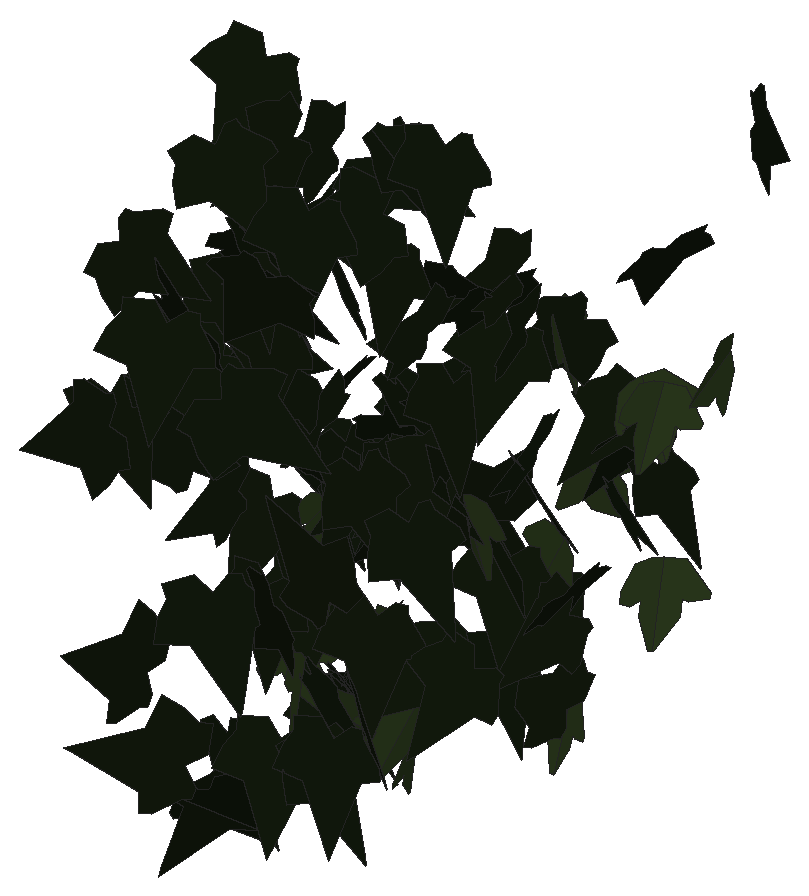
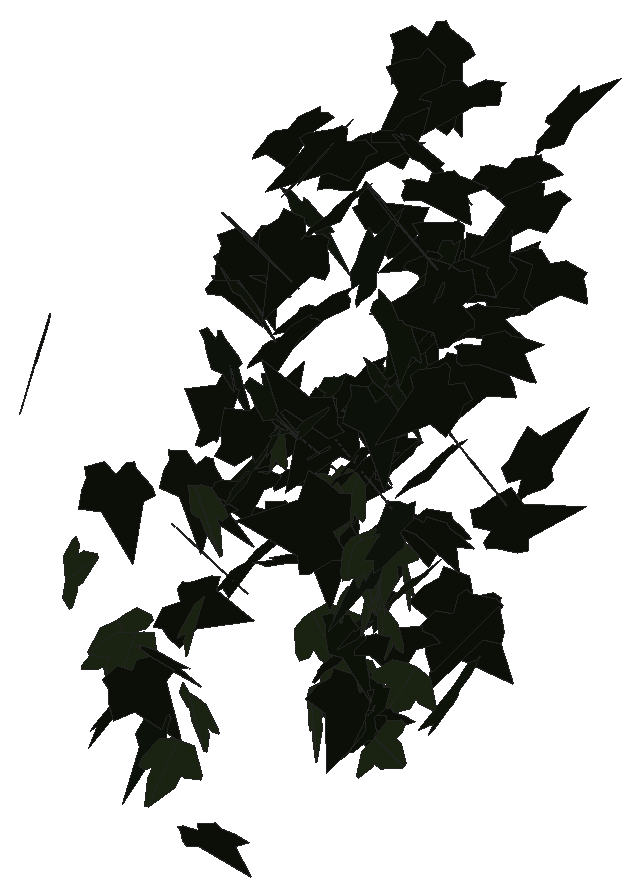
# SketchUp Ruby script. Lengths in inches.
U = 1.inch
M = Sketchup.active_model
def pt(a) = Geom::Point3d.new(a.map { |v| v * U })
def face(e, loops, mat)
  f = e.add_face(loops[0].map { |a| pt(a) })
  loops[1..].each { |l| e.add_face(l.map { |a| pt(a) }).erase! }
  f.material = f.back_material = mat if mat
  f
end
# faces: each face lists its corners as indices into pts; further lists are holes
def faces(e, pts, list, mat = nil) = list.each { |f| face(e, (f[0].is_a?(Array) ? f : [f]).map { |l| l.map { |i| pts[i] } }, mat) }
# xy, xz, yz: faces in a plane at the given z, y or x. An outline is a flat list of corners, or four numbers for a rectangle; further outlines are holes
def ring(l) = l.size == 4 ? [[l[0], l[1]], [l[2], l[1]], [l[2], l[3]], [l[0], l[3]]] : l.each_slice(2).to_a
def flat(e, list, mat, &to3) = list.each { |f| face(e, (f[0].is_a?(Array) ? f : [f]).map { |l| ring(l).map { |u, v| to3.(u, v) } }, mat) }
def xy(e, z, list, mat = nil) = flat(e, list, mat) { |x, y| [x, y, z] }
def xz(e, y, list, mat = nil) = flat(e, list, mat) { |x, z| [x, y, z] }
def yz(e, x, list, mat = nil) = flat(e, list, mat) { |y, z| [x, y, z] }
def lines(e, pts, list) = list.each { |a, b| e.add_line(pt(pts[a]), pt(pts[b])) }
# prism: a flat outline (further loops are holes) pulled along v
def prism(e, loops, v, mat = nil)
  f = face(e, loops, mat); d = Geom::Vector3d.new(v.map { |x| x * U })
  f.pushpull(f.normal.samedirection?(d) ? d.length : -d.length)
end
def box(e, o, s, mat = nil) = prism(e, [[o, [o[0] + s[0], o[1], o[2]], [o[0] + s[0], o[1] + s[1], o[2]], [o[0], o[1] + s[1], o[2]]]], [0, 0, s[2]], mat)
def at(x, y, z, deg = 0) = Geom::Transformation.translation(pt([x, y, z])) * Geom::Transformation.rotation(ORIGIN, Z_AXIS, deg.degrees)
def axes(o, x, y, z) = Geom::Transformation.new([*x, 0, *y, 0, *z, 0, *pt(o).to_a, 1])
def part(name) = M.definitions.add(name)
# library, detail: a bought-in or finely detailed component or shape, given as its bounding box
def library(name, o, s) = part(name).tap { |d| box(d.entities, o, s) }
def detail(e, o, s) = box(e.add_group.entities, o, s)
def put(e, d, t, mat = nil) = e.add_instance(d, t).tap { |i| i.material = mat if mat }
def group(e, t, mat = nil) = e.add_group.tap { |g| g.transformation = t; g.material = mat if mat }.entities
root = M.entities
M.materials.add("efeu1").color = [18, 25, 13]
M.materials.add("efeu2").color = [43, 57, 29]
c1 = part("ivyleaf_9")
p = [[1.54,2.16,1.25],[1.36,2.04,1.19],[-0.21,0.99,0.68],[-0.71,1.11,0.82],[-0.85,0.86,0.67],[-0.8,0.17,0.21],
  [-0.9,-0.01,0.1],[-0.67,-0.16,-0.02],[-0.08,-0.08,-0.05],[-0.03,-0.6,-0.4],[0.65,-0.88,-0.66],[0.83,-0.6,-0.49],
  [1.29,-0.42,-0.43],[1.8125,-0.07,-0.26],[1.21,0.44,0.15]]
faces(c1.entities,p,[[0,1,2,3,4,5,6,7,8,9,10,11,12,13,14]],"efeu1")
c2 = part("ivyleaf_10")
p = [[0,0.5,-0.03],[-0.0625,2.02,-0.43],[-0.19,2.01,-0.46],[-0.54,1.05,-0.29],[-0.52,0.625,-0.18],[-0.83,0.76,-0.28],
  [-1.16,0.64,-0.33],[-1.15,0.33,-0.24],[-0.77,-0.39,0.02],[-0.3,-0.51,0.16],[0.04,-0.48,0.23],[-0.02,2.01,-0.4375],
  [-0.06,2.01,-0.43],[0.04,-0.49,0.23],[0.67,-0.49,0.14],[1.38,0.36,-0.2],[1.375,0.51,-0.24],[0.81,0.65,-0.19],
  [0.62,0.59,-0.15],[0.6,1.09,-0.28],[0.5,1.23,-0.31]]
faces(c2.entities,p,[[0,1,2,3,4,5,6,7,8,9,10],[11,12,0,13,14,15,16,17,18,19,20]],"efeu2")
put(root,c1,axes([629.85,118.33,320.14],[-1.05111,-0.93043,0.08005],[-0.05037,-0.06385,-1.40368],[0.93251,-1.05222,0.0144]))
put(root,c1,axes([629.95,121.9,329.74],[-0.98839,-0.8944,-0.09871],[0.06806,0.0719,-1.33297],[0.89725,-0.9907,-0.00762]))
put(root,c2,axes([629.7,123.79,306.15],[-1.03186,-0.37718,-0.54841],[0.62092,-0.18105,-1.04376],[0.23975,-1.15443,0.34287]))
put(root,c2,axes([630.0625,125.32,303.48],[0.25648,0.92168,-0.76849],[-0.25719,-0.72537,-0.95579],[-1.17215,0.36083,0.04156]))
put(root,c1,axes([629.92,124.72,308.45],[-0.52487,-1.07341,-0.35701],[0.17536,0.3116,-1.1947],[1.11755,-0.55303,0.0198]))
put(root,c1,axes([630.25,121.9,312.72],[-1.12203,-0.49957,-0.40756],[0.40329,0.09442,-1.226],[0.50303,-1.19002,0.07382]))
put(root,c1,axes([629.7,124.1,310.51],[-0.03949,-1.15836,0.48367],[0.26125,-0.4809,-1.13039],[1.2278,0.06507,0.25608]))
put(root,c1,axes([629.79,114.55,325.82],[0.38981,-0.4459,-1.19635],[-0.12214,1.2321,-0.49902],[1.27089,0.25517,0.31899]))
put(root,c1,axes([630.09,120.75,319.09],[0.16006,0.06924,-1.32906],[-0.32833,1.29931,0.02815],[1.28972,0.32218,0.1721]))
put(root,c1,axes([630.9375,122.96,322.99],[-0.20763,1.04748,0.75387],[-0.20421,0.72728,-1.06677],[-1.2743,-0.28722,0.04812]))
put(root,c1,axes([629.64,120.48,304.03],[0.82578,-1.15992,-0.03923],[-0.02272,0.03198,-1.42384],[1.16036,0.82609,0.00004]))
put(root,c1,axes([629.7,120.33,323.08],[0.87461,0.16047,0.98959],[0.83483,0.61055,-0.83683],[-0.55508,1.1711,0.30068]))
put(root,c2,axes([630.15,124.75,309.44],[1.06337,-0.50755,0.41179],[0.44059,-0.02421,-1.16758],[0.48276,1.14006,0.15854]))
put(root,c1,axes([630.91,136.59,303.67],[-1.12475,-0.4794,-0.04315],[0.03909,0.01833,-1.22266],[0.47975,-1.12543,-0.00153]))
put(root,c1,axes([631.46,118.46,315.09],[-1.13617,0.55762,0.10034],[-0.07939,0.06594,-1.2654],[-0.56099,-1.13868,-0.02415]))
put(root,c2,axes([631.16,124.11,312.08],[-0.66363,-1.0746,0.04055],[-0.0351,-0.02598,-1.2629],[1.07479,-0.66436,-0.0162]))
put(root,c1,axes([631.39,117.6875,320.6],[-0.98385,-0.80675,0.37955],[-0.27516,-0.26289,-1.27202],[0.84805,-1.02123,0.02761]))
put(root,c1,axes([630.22,123.89,313.17],[1.06374,-0.68486,0.17281],[0.28329,0.12751,-1.23852],[0.64703,1.07011,0.25817]))
put(root,c2,axes([631.31,124.14,310.46],[-0.9243,0.82505,0.09608],[-0.06849,0.06756,-1.23896],[-0.8278,-0.92682,-0.00478]))
put(root,c1,axes([631.24,124.95,304.01],[-0.66697,-1.02849,-0.18823],[0.13194,0.13869,-1.22533],[1.03722,-0.679,0.03483]))
put(root,c1,axes([631.21,124.12,311.6],[1.05332,-0.1652,-0.6635],[-0.56826,0.46619,-1.01821],[0.38026,1.15428,0.31627]))
put(root,c1,axes([631.51,116.1,322.09],[0.94752,-0.72708,0.58664],[-0.3929,0.44794,1.18977],[-0.8476,-1.02043,0.10428]))
put(root,c1,axes([630.55,125.26,304.54],[0.8076,-0.6856,0.62738],[0.50223,-0.37735,-1.05889],[0.78193,0.95049,0.03215]))
put(root,c1,axes([630.96,112.43,321.17],[-0.5158,-0.64825,-1.06719],[0.73295,0.77762,-0.8266],[1.0109,-0.89457,0.05481]))
put(root,c1,axes([631.53,125,305.17],[0.71702,1.00502,-0.03351],[-0.02036,-0.02664,-1.23458],[-1.00538,0.7173,0.0011]))
put(root,c2,axes([631.74,124.39,312.07],[-0.30232,-1.21917,0.07984],[-0.00639,-0.08067,-1.25603],[1.22177,-0.3021,0.01319]))
put(root,c1,axes([631.92,112.98,310.69],[-0.07155,-0.07773,1.43345],[-0.90642,-1.1105,-0.10546],[1.1132,-0.90922,0.00626]))
put(root,c1,axes([630.89,120.05,323.92],[1.00123,-1.01155,0.16192],[0.10518,-0.12371,-1.42321],[1.01901,1.00667,-0.01219]))
put(root,c1,axes([631.0625,125.2,304.2],[0.80695,-0.89437,0.2562],[0.1472,-0.21213,-1.20417],[0.91862,0.81964,-0.0321]))
put(root,c2,axes([631.78,135.75,314.1875],[-0.42051,1.18964,-0.00915],[0.00364,-0.00842,-1.26177],[-1.18967,-0.42053,-0.00062]))
put(root,c2,axes([631.8,137.46,307.65],[-0.5745,-0.92797,-0.57674],[0.40661,0.42321,-1.08598],[1.01411,-0.69539,0.10871]))
put(root,c1,axes([632.39,135.99,314.27],[-0.05037,-0.10713,-1.26314],[0.05844,-1.26299,0.10479],[-1.26633,-0.05402,0.05508]))
put(root,c1,axes([631.65,118.47,323.52],[-0.62495,-0.85754,-0.91346],[0.6079,0.68505,-1.05901],[1.09555,-0.8693,0.06654]))
put(root,c1,axes([633.02,121.54,327.59],[-1.11631,0.62863,0.29212],[-0.24364,0.1626,-1.28096],[-0.64896,-1.14239,-0.02158]))
put(root,c1,axes([632.76,122.16,317.82],[-0.22972,1.28946,0.09858],[-0.01503,0.09746,-1.30977],[-1.29314,-0.2302,-0.00229]))
put(root,c1,axes([632.84,116.55,304.9],[-0.09098,0.72057,-1.21261],[0.01216,-1.21469,-0.72271],[-1.4105,-0.05695,0.07198]))
put(root,c1,axes([633.11,124.01,307.52],[-0.6434,1.06538,-0.06382],[0.03702,-0.0522,-1.24458],[-1.06665,-0.64444,-0.0047]))
put(root,c1,axes([633.41,113.11,307.55],[-0.46434,-0.17301,1.28913],[-1.22401,-0.40492,-0.49522],[0.44,-1.30901,-0.01719]))
put(root,c1,axes([633.38,119.02,329.18],[-1.30364,0.13098,0.02587],[-0.0265,-0.0049,-1.31018],[-0.13085,-1.30389,0.00753]))
put(root,c1,axes([632.6,120.49,319.2],[-0.3145,-0.86879,0.98752],[-0.16671,-0.98083,-0.91601],[1.30468,-0.33476,0.121]))
put(root,c2,axes([633.06,123.38,305.09],[-1.20093,-0.29196,0.04887],[-0.04994,-0.00147,-1.23587],[0.29178,-1.20193,-0.01036]))
put(root,c2,axes([632.875,123.77,314.48],[-1.16141,0.49647,-0.12463],[0.10957,-0.06074,-1.26301],[-0.50001,-1.1665,0.01272]))
put(root,c1,axes([632.85,115.52,305.27],[0.92996,1.12425,-0.03206],[-0.0205,-0.02464,-1.45902],[-1.12452,0.93018,0.00009]))
put(root,c1,axes([633.85,120.02,317.71],[-0.53939,0.98174,0.63763],[-0.48392,0.45227,-1.10571],[-1.06593,-0.70212,0.17932]))
put(root,c1,axes([633.625,113.4,319.0625],[0.49934,0.07886,1.25223],[-1.23019,0.29591,0.47191],[-0.24683,-1.31524,0.18126]))
put(root,c1,axes([632.8,124.93,306.72],[-0.055,-1.14343,0.47918],[-0.05277,-0.47706,-1.14442],[1.23865,-0.0711,-0.02747]))
put(root,c1,axes([632.875,123.5,315.16],[-0.13164,-1.28628,0.02232],[0.04511,-0.02704,-1.29213],[1.28569,-0.13075,0.04762]))
put(root,c1,axes([632.87,118.84,321.77],[0.00615,-1.28315,0.20176],[0.01801,-0.20166,-1.28306],[1.29879,0.00888,0.01684]))
put(root,c1,axes([633.5,136.28,308],[1.01311,-0.16758,-0.77942],[-0.72651,0.32493,-1.01419],[0.32828,1.23625,0.16091]))
put(root,c1,axes([633.48,112.19,324.92],[-0.65562,-1.16623,-0.35385],[0.14652,0.32346,-1.33756],[1.20989,-0.67114,-0.02977]))
put(root,c1,axes([633.1875,122.4,315.6875],[0.5466,-1.11818,-0.39841],[-0.16331,0.36361,-1.24457],[1.17575,0.57034,0.01235]))
put(root,c1,axes([634.04,123.91,312.18],[0.06649,1.23552,-0.18182],[0.03052,-0.18363,-1.23666],[-1.24845,0.06131,-0.03992]))
put(root,c1,axes([634.09,136.44,311.53],[-1.19984,-0.29103,-0.13396],[0.19017,-0.22908,-1.20566],[0.25783,-1.18536,0.26589]))
put(root,c1,axes([632.53,125.73,313.32],[0.98211,-0.15036,1.11304],[1.09701,-0.18875,-0.99346],[0.24093,1.47234,-0.01369]))
put(root,c2,axes([634.05,124.09,314.1875],[1.0702,-0.45992,-0.50399],[-0.34422,0.44551,-1.13749],[0.5891,1.09583,0.25092]))
put(root,c2,axes([633.33,124.16,307.99],[0.38365,-0.89436,0.77072],[0.76379,-0.42994,-0.87912],[0.90028,0.74588,0.41739]))
put(root,c2,axes([633.7,119.11,308.51],[0.86887,-0.88769,0.20514],[0.24135,-0.04909,-1.23465],[0.87854,0.89141,0.1363]))
put(root,c1,axes([633.26,115.29,330.37],[0.06426,-1.04309,-0.8488],[0.32117,0.83708,-1.00438],[1.30589,-0.15454,0.28879]))
put(root,c1,axes([634.45,136.76,310.36],[-0.28646,0.88755,-0.82327],[-0.01538,-0.8486,-0.90951],[-1.21049,-0.19925,0.20638]))
put(root,c1,axes([633.4,120.41,307.6],[1.08114,-0.66884,-0.30097],[-0.1992,0.24818,-1.26709],[0.70586,1.09446,0.1034]))
put(root,c1,axes([634.73,122.07,315.1],[-1.17873,0.5102,-0.00308],[0.00207,-0.00296,-1.2844],[-0.5102,-1.17873,0.00189]))
put(root,c1,axes([633.59,117.63,312.44],[0.01918,-1.29717,0.25437],[0.09259,-0.25246,-1.29438],[1.31863,0.03659,0.08719]))
put(root,c1,axes([633.51,123.92,313.35],[0.2741,-1.19673,0.34469],[0.19792,-0.30659,-1.22186],[1.22955,0.31614,0.11984]))
put(root,c2,axes([634.26,124.63,303.7],[0.42762,-1.12991,-0.3278],[-0.03792,0.33537,-1.20545],[1.17589,0.42172,0.08034]))
put(root,c1,axes([635.29,123.45,313.48],[-0.43888,0.61683,1.00301],[-0.61973,0.78917,-0.75649],[-1.00122,-0.75885,0.02858]))
put(root,c1,axes([633.55,118.66,317.24],[1.19075,-0.32832,0.32068],[0.34898,0.06861,-1.22557],[0.29807,1.23126,0.15381]))
put(root,c1,axes([634.82,120.61,322.68],[0.42478,-1.11543,0.79685],[-0.2969,0.73957,1.19352],[-1.33828,-0.51812,-0.01186]))
put(root,c1,axes([634.62,121.09,315.47],[-1.10663,0.05032,-0.70148],[0.69294,-0.14542,-1.10359],[-0.12015,-1.30213,0.09614]))
put(root,c1,axes([634.36,123.07,316.97],[0.94932,0.85928,0.09773],[0.06493,0.07389,-1.28041],[-0.86238,0.95147,0.01118]))
put(root,c2,axes([634.6,136.82,311.89],[0.56606,1.07405,0.2793],[0.08691,0.26967,-1.21315],[-1.10636,0.57071,0.0476]))
put(root,c1,axes([635.05,124.3,314.98],[-0.35719,-1.20418,0.11684],[0.00889,-0.12443,-1.25528],[1.2098,-0.35461,0.04372]))
put(root,c1,axes([635.33,106.64,324.12],[0.20822,-0.94646,-0.9854],[0.3729,-0.91957,0.96203],[-1.31444,-0.4108,0.11683]))
put(root,c1,axes([634.56,123.52,317.9375],[0.93496,-0.88647,-0.04828],[0.13282,0.209,-1.2653],[0.87779,0.91258,0.24288]))
put(root,c2,axes([635.77,122.41,306.03],[-0.59553,-0.97457,0.53729],[-0.20555,-0.50257,-1.13942],[1.09371,-0.6251,0.07841]))
put(root,c1,axes([634.99,137.02,309.04],[0.51399,-1.05442,-0.41332],[-0.14528,0.38876,-1.17242],[1.12318,0.53281,0.0375]))
put(root,c1,axes([635.11,112.77,314.77],[-0.58043,-0.88967,-0.93929],[0.48572,0.80432,-1.06199],[1.1991,-0.75646,-0.02449]))
put(root,c2,axes([635.52,136.37,312.16],[0.57861,1.01382,-0.44515],[-0.22003,-0.38697,-1.16731],[-1.08516,0.61903,-0.00067]))
put(root,c1,axes([635.08,123.82,316.74],[-0.59901,0.21651,1.10848],[1.03959,-0.3847,0.63692],[0.44142,1.19981,0.0042]))
put(root,c1,axes([634.76,113.86,321.72],[0.35472,-0.54715,-1.30549],[0.57702,1.28486,-0.38172],[1.29257,-0.42342,0.52867]))
put(root,c1,axes([636.375,123.64,316],[-1.24976,0.19654,-0.06045],[0.03188,-0.18269,-1.25292],[-0.20314,-1.23782,0.17532]))
put(root,c1,axes([635.86,115.37,308.26],[-0.86375,-0.86096,-0.59236],[0.45594,0.38105,-1.21866],[0.94035,-0.97558,0.04677]))
put(root,c1,axes([636.52,135.4375,318.76],[-0.03754,1.22839,-0.38138],[-0.03869,-0.38245,-1.22802],[-1.28565,-0.02435,0.04809]))
put(root,c1,axes([635.9375,116.85,328.0625],[-0.28988,-1.37156,-0.16549],[0.01378,0.16622,-1.40171],[1.38144,-0.28947,-0.02075]))
put(root,c1,axes([636.85,119.51,327.24],[-0.00469,-0.8214,-1.09659],[-0.01841,-1.09646,0.82139],[-1.36999,0.01754,-0.00728]))
put(root,c1,axes([636.06,119.53,316.84],[0.26617,-1.17217,-0.62284],[-0.15215,0.60411,-1.20195],[1.31862,0.30632,-0.01297]))
put(root,c1,axes([637.3125,122,316.27],[-1.25456,-0.09063,0.16456],[-0.16407,-0.01264,-1.25783],[0.0915,-1.26525,0.00078]))
put(root,c1,axes([636.43,119.93,311.1875],[-0.29602,-1.32053,-0.25073],[0.02089,0.25219,-1.35287],[1.34396,-0.29478,-0.0342]))
put(root,c1,axes([636.14,120.27,328.81],[0.40051,-0.43282,-1.2469],[0.13546,1.30964,-0.41109],[1.31292,-0.00308,0.42279]))
put(root,c1,axes([636.16,121.24,329.02],[0.79281,-1.05829,-0.35194],[-0.07844,0.37782,-1.31281],[1.11251,0.7808,0.15824]))
put(root,c1,axes([637.78,123.54,317.53],[-0.89822,0.87982,-0.14322],[-0.11884,-0.3197,-1.21864],[-0.88345,-0.85153,0.30955]))
put(root,c1,axes([636.67,120.52,325.23],[-0.07865,-1.28965,0.34276],[0.06168,-0.3465,-1.28957],[1.333,-0.06005,0.0799]))
put(root,c1,axes([637.59,122.93,308.88],[-1.07031,-0.59375,0.4291],[-0.11526,-0.61377,-1.13677],[0.72345,-0.97621,0.45373]))
put(root,c1,axes([638,112.35,315.6],[0.50833,0.08596,-1.26753],[-1.26481,-0.09413,-0.51362],[-0.11946,1.36241,0.04449]))
put(root,c1,axes([637.24,121.6,324.26],[1.17262,0.55782,-0.30408],[-0.30958,-0.0557,-1.29604],[-0.55478,1.21012,0.08051]))
put(root,c1,axes([637.35,123.8125,314.97],[-0.34022,-0.28023,1.19531],[-0.01508,-1.23931,-0.29484],[1.22762,-0.09289,0.32764]))
put(root,c2,axes([637.43,128.87,304.4],[1.15558,-0.47439,0.09499],[0.09233,-0.02523,-1.24911],[0.47492,1.1592,0.01169]))
put(root,c1,axes([637.26,112.29,327.74],[1.26967,0.4718,0.15703],[0.14515,0.06021,-1.35448],[-0.47559,1.27793,0.00584]))
put(root,c2,axes([637.87,136.97,314.19],[-0.09906,0.22167,-1.23551],[-0.03414,-1.23937,-0.21963],[-1.25477,0.01622,0.10352]))
put(root,c1,axes([638.65,111.18,329],[0.57628,0.60588,-1.21717],[-0.95096,-0.76522,-0.83115],[-0.97173,1.10817,0.09154]))
put(root,c1,axes([638.34,123.62,314.29],[0.47976,0.42525,1.37572],[-1.16772,-0.73357,0.63398],[0.84254,-1.25883,0.0953]))
put(root,c1,axes([637.76,122.44,319.58],[0.01369,-1.28329,-0.10753],[-0.00453,0.10748,-1.28336],[1.28778,0.01402,-0.00337]))
put(root,c2,axes([638.18,122.79,314.86],[-1.19579,0.34877,-0.24208],[0.1979,-0.18222,-1.24008],[-0.37561,-1.20636,0.11732]))
put(root,c1,axes([637.37,117.78,309.08],[0.47015,-0.15022,-1.34261],[1.32215,-0.24099,0.48995],[-0.27764,-1.40199,0.05964]))
put(root,c1,axes([638.14,121.46,329.33],[-0.10375,-1.33603,-0.1816],[-0.01153,0.18301,-1.33981],[1.34827,-0.10124,-0.02543]))
put(root,c1,axes([639.46,118.75,323.875],[-0.76288,0.98086,0.37583],[-0.36712,0.18622,-1.2312],[-0.98415,-0.82979,0.16795]))
put(root,c1,axes([637.99,124.33,313.69],[0.53838,-1.1048,0.28439],[0.13965,-0.24828,-1.22889],[1.13223,0.55596,0.01634]))
put(root,c2,axes([638.74,132.4375,308.21],[0.7446,1.00185,-0.18775],[-0.13055,-0.13686,-1.24804],[-1.0109,0.75561,0.02288]))
put(root,c1,axes([639.33,122.54,323.77],[-0.03197,1.19856,-0.54827],[-0.01909,-0.54879,-1.1986],[-1.31787,-0.02113,0.03066]))
put(root,c1,axes([638.49,124.07,308.86],[0.27329,-1.23369,-0.12422],[-0.0213,0.12251,-1.26359],[1.23975,0.27406,0.00568]))
put(root,c1,axes([639.91,122.85,324.55],[-1.1121,0.62478,0.25885],[-0.28307,0.0224,-1.27023],[-0.61418,-1.1416,0.11674]))
put(root,c1,axes([638.43,114.1,309.32],[0.57611,-1.23103,-0.41821],[-0.04868,0.43668,-1.35247],[1.29922,0.56224,0.13476]))
put(root,c1,axes([638.98,123.93,312.64],[-0.44122,-1.16685,-0.26044],[0.08979,0.24448,-1.24748],[1.19219,-0.45026,-0.00243]))
put(root,c2,axes([639.47,125.79,312.46],[1.05379,-0.41487,-0.54309],[-0.43371,0.36539,-1.12068],[0.52817,1.12779,0.1633]))
put(root,c1,axes([639.53,121.14,309.78],[-1.11583,-0.60101,-0.02105],[0.01801,0.01095,-1.2674],[0.60111,-1.11598,-0.0011]))
put(root,c1,axes([638.97,114.41,309.75],[-0.18087,-1.35009,-0.11912],[0.01541,0.11812,-1.36215],[1.35525,-0.18153,-0.00041]))
put(root,c1,axes([640.14,123.1,322.46],[-0.98491,0.8125,0.05806],[-0.04792,0.03314,-1.27678],[-0.81316,-0.98606,0.00492]))
put(root,c1,axes([639.6875,123.07,321.89],[-0.92801,-0.8262,-0.34702],[0.28891,0.19704,-1.24175],[0.84826,-0.97098,0.04329]))
put(root,c1,axes([640.29,135.67,324.84],[0.54041,-0.09807,-1.18016],[-1.03159,0.59806,-0.52208],[0.58155,1.15201,0.17056]))
put(root,c1,axes([641.11,122.65,318.1875],[-0.81115,0.99047,0.0013],[0.03146,0.02744,-1.27955],[-0.98997,-0.81068,-0.04172]))
put(root,c1,axes([641.27,124.06,311.21],[-1.25741,-0.19818,0.02701],[-0.02703,-0.00198,-1.27293],[0.19818,-1.2577,-0.00225]))
put(root,c1,axes([639.9,124.05,315.68],[0.54401,-0.71336,0.89818],[0.54269,-0.71568,-0.89712],[1.01049,0.76842,-0.00173]))
put(root,c1,axes([641.8,123.3125,308.22],[-0.65155,0.79803,0.75259],[-0.68545,0.38719,-1.004],[-0.85639,-0.91706,0.23101]))
put(root,c1,axes([641.8,110.49,318.125],[0.19689,0.0387,1.38181],[-1.07363,0.88348,0.12824],[-0.87075,-1.08057,0.15433]))
put(root,c1,axes([640.44,116.74,317.6],[0.25553,-1.25168,-0.58974],[0.03744,0.60575,-1.26943],[1.38315,0.21485,0.14332]))
put(root,c1,axes([641.53,123.72,312.3],[-0.11709,1.27595,-0.00124],[-0.00019,-0.00126,-1.28132],[-1.27595,-0.11709,0.0003]))
